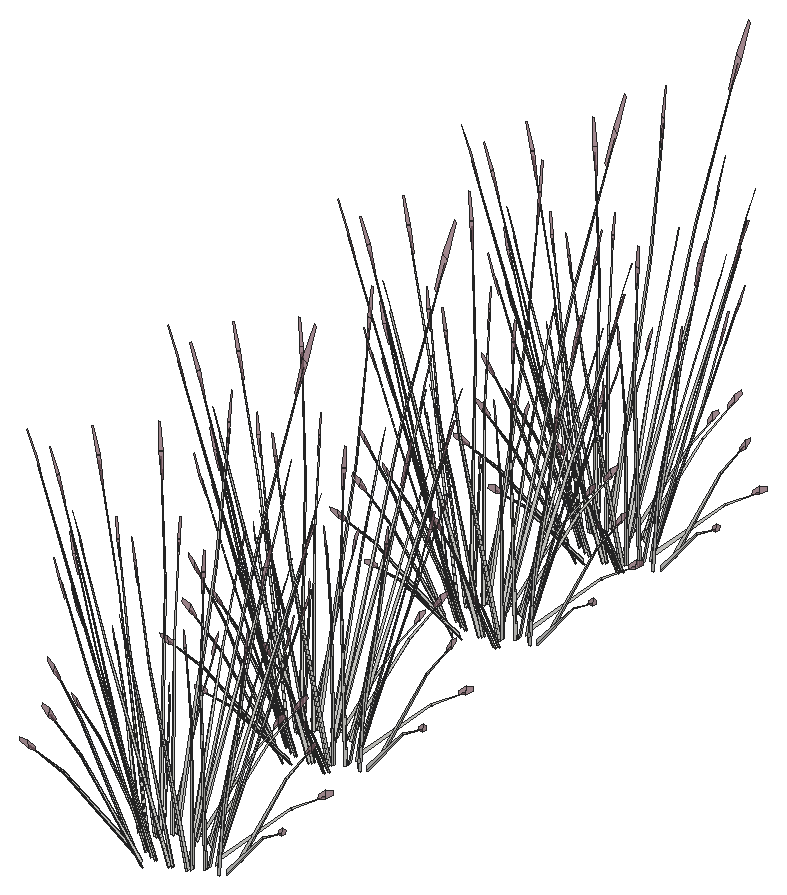
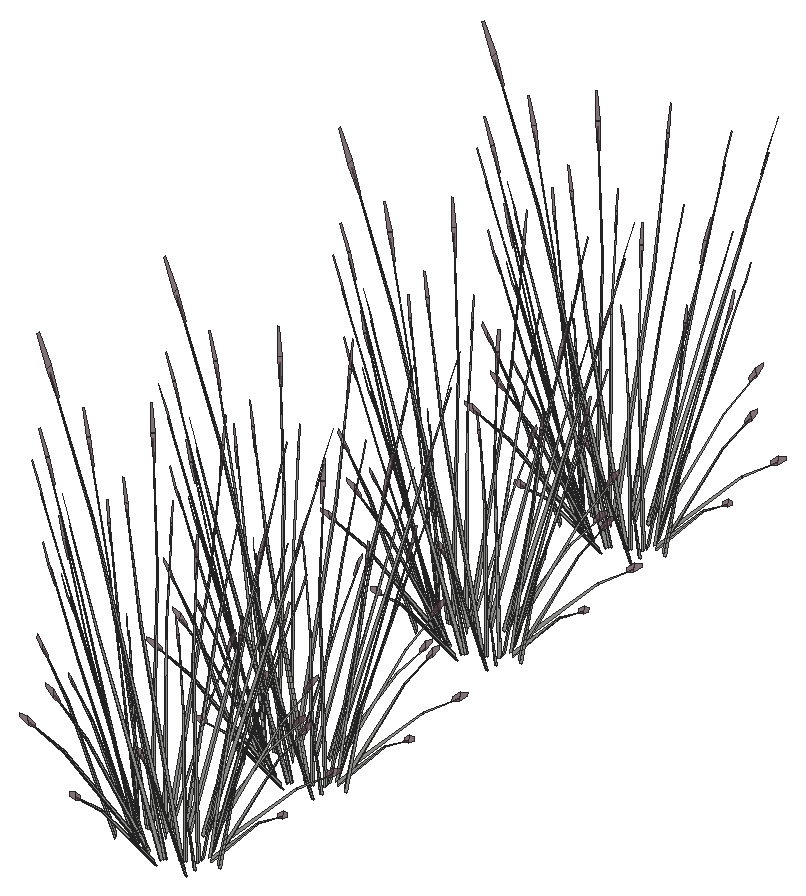
# SketchUp Ruby script. Lengths in inches.
U = 1.inch
M = Sketchup.active_model
def pt(a) = Geom::Point3d.new(a.map { |v| v * U })
def face(e, loops, mat)
  f = e.add_face(loops[0].map { |a| pt(a) })
  loops[1..].each { |l| e.add_face(l.map { |a| pt(a) }).erase! }
  f.material = f.back_material = mat if mat
  f
end
# faces: each face lists its corners as indices into pts; further lists are holes
def faces(e, pts, list, mat = nil) = list.each { |f| face(e, (f[0].is_a?(Array) ? f : [f]).map { |l| l.map { |i| pts[i] } }, mat) }
# xy, xz, yz: faces in a plane at the given z, y or x. An outline is a flat list of corners, or four numbers for a rectangle; further outlines are holes
def ring(l) = l.size == 4 ? [[l[0], l[1]], [l[2], l[1]], [l[2], l[3]], [l[0], l[3]]] : l.each_slice(2).to_a
def flat(e, list, mat, &to3) = list.each { |f| face(e, (f[0].is_a?(Array) ? f : [f]).map { |l| ring(l).map { |u, v| to3.(u, v) } }, mat) }
def xy(e, z, list, mat = nil) = flat(e, list, mat) { |x, y| [x, y, z] }
def xz(e, y, list, mat = nil) = flat(e, list, mat) { |x, z| [x, y, z] }
def yz(e, x, list, mat = nil) = flat(e, list, mat) { |y, z| [x, y, z] }
def lines(e, pts, list) = list.each { |a, b| e.add_line(pt(pts[a]), pt(pts[b])) }
# prism: a flat outline (further loops are holes) pulled along v
def prism(e, loops, v, mat = nil)
  f = face(e, loops, mat); d = Geom::Vector3d.new(v.map { |x| x * U })
  f.pushpull(f.normal.samedirection?(d) ? d.length : -d.length)
end
def box(e, o, s, mat = nil) = prism(e, [[o, [o[0] + s[0], o[1], o[2]], [o[0] + s[0], o[1] + s[1], o[2]], [o[0], o[1] + s[1], o[2]]]], [0, 0, s[2]], mat)
def at(x, y, z, deg = 0) = Geom::Transformation.translation(pt([x, y, z])) * Geom::Transformation.rotation(ORIGIN, Z_AXIS, deg.degrees)
def axes(o, x, y, z) = Geom::Transformation.new([*x, 0, *y, 0, *z, 0, *pt(o).to_a, 1])
def part(name) = M.definitions.add(name)
# library, detail: a bought-in or finely detailed component or shape, given as its bounding box
def library(name, o, s) = part(name).tap { |d| box(d.entities, o, s) }
def detail(e, o, s) = box(e.add_group.entities, o, s)
def put(e, d, t, mat = nil) = e.add_instance(d, t).tap { |i| i.material = mat if mat }
def group(e, t, mat = nil) = e.add_group.tap { |g| g.transformation = t; g.material = mat if mat }.entities
root = M.entities
M.materials.add("LightPink_Translucent").color = [144, 107, 117]
M.materials["LightPink_Translucent"].alpha = 0.75
c1 = part("blade")
p = [[2.15,0.21,22],[0,0.17,0],[0.09,0.45,0],[2.18,0.31,22],[2.29,0.31,22],[0.38,0.45,0],
  [2.48,0.24,33],[2.49,0.24,33],[2.48,0.22,33]]
faces(c1.entities,p,[[0,1,2,3],[4,5,2,3],[6,3,4,7],[8,0,3,6]])
c2 = part("seeds")
p = [[0.3,-0.1,1.38],[-0.01,-0.03,1.59],[-0.01,-0.03,0.03],[0.14,-0.07,-0.07],[0.29,-0.03,3],[0.15,0.01,3.11]]
faces(c2.entities,p,[[0,1,2,3],[1,0,4,5]],"LightPink_Translucent")
c3 = part("blade with seeds")
put(c3.entities,c1,at(0,0,0))
put(c3.entities,c2,axes([2.4,0.25,30.99],[1.5799,-0.05474,1.17369],[-0.12525,1.92788,0.29478],[-0.07173,-0.02425,1.56792]))
put(root,c3,axes([407.79,166.14,259.71],[-0.01417,0.07324,1.77383],[-0.6991,0.2658,-0.16761],[-0.20573,-0.13587,0.31391]))
put(root,c3,axes([409.76,167.74,260.03],[-0.74352,0.28449,-0.1216],[-0.36538,-0.50492,-0.67495],[-0.0981,-0.21277,1.02557]))
put(root,c3,axes([411.31,168.38,260.03],[-0.83505,-0.03027,-0.1216],[0.02282,-0.57322,-0.67495],[0.05801,-0.22077,1.02557]))
put(root,c3,axes([409.75,167.51,259.73],[0.55987,-0.20767,0.0643],[0.27403,0.37869,0.50621],[-0.05407,-0.16693,0.77189]))
put(root,c3,axes([407.83,167.57,259.73],[0.34533,-0.38816,0.0643],[0.49176,0.22599,0.50621],[-0.15898,-0.12445,0.77189]))
put(root,c3,axes([407.98,167.53,260.43],[-0.50709,0.58578,-0.13619],[-0.73436,-0.33748,-0.75594],[-0.25527,-0.1655,1.14864]))
put(root,c3,axes([411.45,168.18,259.73],[0.62439,0.02847,0.0643],[-0.01712,0.42991,0.50621],[0.06534,-0.16468,0.77189]))
put(root,c3,axes([406.04,167.36,259.72],[-0.16348,-0.00431,1.74944],[-0.52047,0.43131,-0.27667],[-0.2777,-0.08813,0.14031]))
put(root,c3,axes([412.22,169.51,260.03],[-0.70283,-0.33692,-0.1216],[0.40491,-0.48793,-0.67495],[0.19857,-0.16961,1.02557]))
put(root,c3,axes([413.95,169.36,259.71],[-0.09924,-0.00464,1.77383],[-0.4121,-0.49725,-0.16761],[0.1655,-0.1635,0.31391]))
put(root,c3,axes([406.21,168.33,259.73],[0.03826,-0.46465,0.0643],[0.57772,0.01274,0.50621],[-0.2213,-0.04862,0.77189]))
put(root,c3,axes([412.47,169.38,259.73],[0.52161,0.25698,0.0643],[-0.30368,0.36595,0.50621],[0.16723,-0.11831,0.77189]))
put(root,c3,axes([414.32,169.96,259.72],[0.10543,-0.09307,1.74944],[-0.13495,-0.57092,-0.27667],[0.26455,-0.10825,0.14031]))
put(root,c3,axes([405.41,167.73,259.71],[0.05633,0.06098,1.77383],[-0.27155,0.54815,-0.16761],[-0.27501,0.00397,0.31391]))
put(root,c3,axes([406.48,168.4375,260.03],[-0.04068,0.62141,-0.1216],[-0.77029,-0.01698,-0.67495],[-0.29667,-0.04317,1.02557]))
put(root,c3,axes([412.24,170.82,260.03],[-0.38229,-0.5533,-0.1216],[0.6785,-0.2719,-0.67495],[0.28593,-0.073,1.02557]))
put(root,c3,axes([405.31,169.6,259.73],[-0.27906,-0.41663,0.0643],[0.50888,-0.20393,0.50621],[-0.22432,0.04024,0.77189]))
put(root,c3,axes([412.55,170.8125,259.73],[0.27906,0.41663,0.0643],[-0.50888,0.20393,0.50621],[0.22432,-0.04024,0.77189]))
put(root,c3,axes([413.76,172.47,259.71],[-0.0687,-0.05349,1.77383],[0.15029,-0.57341,-0.16761],[0.27062,-0.03664,0.31391]))
put(root,c3,axes([404.82,170.14,259.72],[-0.12407,0.07933,1.74944],[0.01055,0.57963,-0.27667],[-0.2844,0.07538,0.14031]))
put(root,c3,axes([405.62,169.59,260.03],[0.38229,0.5533,-0.1216],[-0.6785,0.2719,-0.67495],[-0.28593,0.073,1.02557]))
put(root,c3,axes([411.39,171.97,260.03],[0.04068,-0.62141,-0.1216],[0.77029,0.01698,-0.67495],[0.29667,0.04317,1.02557]))
put(root,c3,axes([412.06,171.6,259.72],[0.16299,-0.01033,1.74944],[0.44707,-0.47471,-0.27667],[0.28992,0.06266,0.14031]))
put(root,c3,axes([405.39,171.03,259.73],[-0.52161,-0.25698,0.0643],[0.30368,-0.36595,0.50621],[-0.16723,0.11831,0.77189]))
put(root,c3,axes([403.44,170.73,259.71],[0.09697,0.01639,1.77383],[0.29997,0.53988,-0.16761],[-0.1985,0.1417,0.31391]))
put(root,c3,axes([411.66,172.08,259.73],[-0.03826,0.46465,0.0643],[-0.57772,-0.01274,0.50621],[0.2213,0.04862,0.77189]))
put(root,c3,axes([410.38,169.5625,259.47],[-0.65655,-0.31748,1.38283],[0.69326,-0.49431,0.59665],[0.21183,0.29789,1.33663]))
put(root,c3,axes([405.65,170.9,260.03],[0.70283,0.33692,-0.1216],[-0.40491,0.48793,-0.67495],[-0.19857,0.16961,1.02557]))
put(root,c3,axes([409.87,172.65,260.03],[0.45276,-0.52302,-0.1216],[0.65568,0.30132,-0.67495],[0.22792,0.14777,1.02557]))
put(root,c3,axes([409.28,173.08,259.71],[0.00225,-0.07398,1.77383],[0.65113,-0.32638,-0.16761],[0.22617,0.1165,0.31391]))
put(root,c3,axes([406.42,172.23,259.73],[-0.62439,-0.02847,0.0643],[0.01712,-0.42991,0.50621],[-0.06534,0.16468,0.77189]))
put(root,c3,axes([410.04,172.84,259.73],[-0.34533,0.38816,0.0643],[-0.49176,-0.22599,0.50621],[0.15898,0.12445,0.77189]))
put(root,c3,axes([408.12,172.9,259.73],[-0.55987,0.20767,0.0643],[-0.27403,-0.37869,0.50621],[0.05407,0.16693,0.77189]))
put(root,c3,axes([404.84,172.3,259.72],[-0.01889,0.12092,1.74944],[0.53598,0.42065,-0.27667],[-0.14032,0.19892,0.14031]))
put(root,c3,axes([406.56,172.03,260.4],[0.83505,0.03027,-0.13498],[-0.02282,0.57322,-0.74919],[-0.05801,0.22077,1.13838]))
put(root,c3,axes([408.1,172.67,260.03],[0.74352,-0.28449,-0.1216],[0.36538,0.50492,-0.67495],[0.0981,0.21277,1.02557]))
put(root,c3,axes([404.78,173.54,259.71],[0.0862,-0.03689,1.77383],[0.71245,0.24539,-0.16761],[-0.01674,0.20431,0.31391]))
put(root,c3,axes([407.93,173.8,259.72],[0.09631,0.0984,1.74944],[0.77725,0.03866,-0.27667],[0.07816,0.217,0.14031]))
put(root,c3,axes([406.5625,188.55,259.72],[-0.11621,-0.08567,1.74944],[-0.77555,0.05431,-0.27667],[-0.12378,-0.20491,0.14031]))
put(root,c3,axes([410.05,189.6,259.72],[-0.00733,-0.12161,1.74944],[-0.61946,-0.35147,-0.27667],[0.09577,-0.21306,0.14031]))
put(root,c3,axes([409.88,189.16,259.71],[-0.07716,0.04667,1.77383],[-0.75601,-0.15746,-0.16761],[-0.02737,-0.20368,0.31391]))
put(root,c3,axes([405.77,188.27,259.71],[-0.01417,0.07324,1.77383],[-0.6991,0.2658,-0.16761],[-0.20573,-0.13587,0.31391]))
put(root,c3,axes([407.74,189.87,260.03],[-0.74352,0.28449,-0.1216],[-0.36538,-0.50492,-0.67495],[-0.0981,-0.21277,1.02557]))
put(root,c3,axes([409.29,190.51,260.03],[-0.83505,-0.03027,-0.1216],[0.02282,-0.57322,-0.67495],[0.05801,-0.22077,1.02557]))
put(root,c3,axes([407.73,189.64,259.73],[0.55987,-0.20767,0.0643],[0.27403,0.37869,0.50621],[-0.05407,-0.16693,0.77189]))
put(root,c3,axes([405.81,189.7,259.73],[0.34533,-0.38816,0.0643],[0.49176,0.22599,0.50621],[-0.15898,-0.12445,0.77189]))
put(root,c3,axes([405.96,189.66,260.43],[-0.50709,0.58578,-0.13619],[-0.73436,-0.33748,-0.75594],[-0.25527,-0.1655,1.14864]))
put(root,c3,axes([409.43,190.31,259.73],[0.62439,0.02847,0.0643],[-0.01712,0.42991,0.50621],[0.06534,-0.16468,0.77189]))
put(root,c3,axes([404.02,189.49,259.72],[-0.16348,-0.00431,1.74944],[-0.52047,0.43131,-0.27667],[-0.2777,-0.08813,0.14031]))
put(root,c3,axes([410.2,191.64,260.03],[-0.70283,-0.33692,-0.1216],[0.40491,-0.48793,-0.67495],[0.19857,-0.16961,1.02557]))
put(root,c3,axes([411.93,191.49,259.71],[-0.09924,-0.00464,1.77383],[-0.4121,-0.49725,-0.16761],[0.1655,-0.1635,0.31391]))
put(root,c3,axes([404.1875,190.47,259.73],[0.03826,-0.46465,0.0643],[0.57772,0.01274,0.50621],[-0.2213,-0.04862,0.77189]))
put(root,c3,axes([410.45,191.51,259.73],[0.52161,0.25698,0.0643],[-0.30368,0.36595,0.50621],[0.16723,-0.11831,0.77189]))
put(root,c3,axes([412.3,192.09,259.72],[0.10543,-0.09307,1.74944],[-0.13495,-0.57092,-0.27667],[0.26455,-0.10825,0.14031]))
put(root,c3,axes([403.39,189.86,259.71],[0.05633,0.06098,1.77383],[-0.27155,0.54815,-0.16761],[-0.27501,0.00397,0.31391]))
put(root,c3,axes([404.46,190.57,260.03],[-0.04068,0.62141,-0.1216],[-0.77029,-0.01698,-0.67495],[-0.29667,-0.04317,1.02557]))
put(root,c3,axes([410.23,192.95,260.03],[-0.38229,-0.5533,-0.1216],[0.6785,-0.2719,-0.67495],[0.28593,-0.073,1.02557]))
put(root,c3,axes([403.3,191.73,259.73],[-0.27906,-0.41663,0.0643],[0.50888,-0.20393,0.50621],[-0.22432,0.04024,0.77189]))
put(root,c3,axes([410.53,192.94,259.73],[0.27906,0.41663,0.0643],[-0.50888,0.20393,0.50621],[0.22432,-0.04024,0.77189]))
put(root,c3,axes([411.75,194.6,259.71],[-0.0687,-0.05349,1.77383],[0.15029,-0.57341,-0.16761],[0.27062,-0.03664,0.31391]))
put(root,c3,axes([402.8,192.27,259.72],[-0.12407,0.07933,1.74944],[0.01055,0.57963,-0.27667],[-0.2844,0.07538,0.14031]))
put(root,c3,axes([403.6,191.72,260.03],[0.38229,0.5533,-0.1216],[-0.6785,0.2719,-0.67495],[-0.28593,0.073,1.02557]))
put(root,c3,axes([409.37,194.1,260.03],[0.04068,-0.62141,-0.1216],[0.77029,0.01698,-0.67495],[0.29667,0.04317,1.02557]))
put(root,c3,axes([410.04,193.73,259.72],[0.16299,-0.01033,1.74944],[0.44707,-0.47471,-0.27667],[0.28992,0.06266,0.14031]))
put(root,c3,axes([403.375,193.16,259.73],[-0.52161,-0.25698,0.0643],[0.30368,-0.36595,0.50621],[-0.16723,0.11831,0.77189]))
put(root,c3,axes([401.43,192.86,259.71],[0.09697,0.01639,1.77383],[0.29997,0.53988,-0.16761],[-0.1985,0.1417,0.31391]))
put(root,c3,axes([409.64,194.21,259.73],[-0.03826,0.46465,0.0643],[-0.57772,-0.01274,0.50621],[0.2213,0.04862,0.77189]))
put(root,c3,axes([408.36,191.69,259.47],[-0.65655,-0.31748,1.38283],[0.69326,-0.49431,0.59665],[0.21183,0.29789,1.33663]))
put(root,c3,axes([403.63,193.03,260.03],[0.70283,0.33692,-0.1216],[-0.40491,0.48793,-0.67495],[-0.19857,0.16961,1.02557]))
put(root,c3,axes([407.85,194.78,260.03],[0.45276,-0.52302,-0.1216],[0.65568,0.30132,-0.67495],[0.22792,0.14777,1.02557]))
put(root,c3,axes([407.26,195.21,259.71],[0.00225,-0.07398,1.77383],[0.65113,-0.32638,-0.16761],[0.22617,0.1165,0.31391]))
put(root,c3,axes([404.4,194.37,259.73],[-0.62439,-0.02847,0.0643],[0.01712,-0.42991,0.50621],[-0.06534,0.16468,0.77189]))
put(root,c3,axes([408.02,194.97,259.73],[-0.34533,0.38816,0.0643],[-0.49176,-0.22599,0.50621],[0.15898,0.12445,0.77189]))
put(root,c3,axes([406.1,195.03,259.73],[-0.55987,0.20767,0.0643],[-0.27403,-0.37869,0.50621],[0.05407,0.16693,0.77189]))
put(root,c3,axes([402.82,194.43,259.72],[-0.01889,0.12092,1.74944],[0.53598,0.42065,-0.27667],[-0.14032,0.19892,0.14031]))
put(root,c3,axes([404.54,194.16,260.4],[0.83505,0.03027,-0.13498],[-0.02282,0.57322,-0.74919],[-0.05801,0.22077,1.13838]))
put(root,c3,axes([406.08,194.8,260.03],[0.74352,-0.28449,-0.1216],[0.36538,0.50492,-0.67495],[0.0981,0.21277,1.02557]))
put(root,c3,axes([402.76,195.67,259.71],[0.0862,-0.03689,1.77383],[0.71245,0.24539,-0.16761],[-0.01674,0.20431,0.31391]))
put(root,c3,axes([405.91,195.93,259.72],[0.09631,0.0984,1.74944],[0.77725,0.03866,-0.27667],[0.07816,0.217,0.14031]))
put(root,c3,axes([404.16,215.3,259.72],[-0.11621,-0.08567,1.74944],[-0.77555,0.05431,-0.27667],[-0.12378,-0.20491,0.14031]))
put(root,c3,axes([407.64,216.35,259.72],[-0.00733,-0.12161,1.74944],[-0.61946,-0.35147,-0.27667],[0.09577,-0.21306,0.14031]))
put(root,c3,axes([407.48,215.92,259.71],[-0.07716,0.04667,1.77383],[-0.75601,-0.15746,-0.16761],[-0.02737,-0.20368,0.31391]))
put(root,c3,axes([403.37,215.02,259.71],[-0.01417,0.07324,1.77383],[-0.6991,0.2658,-0.16761],[-0.20573,-0.13587,0.31391]))
put(root,c3,axes([405.34,216.625,260.03],[-0.74352,0.28449,-0.1216],[-0.36538,-0.50492,-0.67495],[-0.0981,-0.21277,1.02557]))
put(root,c3,axes([406.89,217.26,260.03],[-0.83505,-0.03027,-0.1216],[0.02282,-0.57322,-0.67495],[0.05801,-0.22077,1.02557]))
put(root,c3,axes([405.32,216.4,259.73],[0.55987,-0.20767,0.0643],[0.27403,0.37869,0.50621],[-0.05407,-0.16693,0.77189]))
put(root,c3,axes([403.41,216.46,259.73],[0.34533,-0.38816,0.0643],[0.49176,0.22599,0.50621],[-0.15898,-0.12445,0.77189]))
put(root,c3,axes([403.5625,216.42,260.43],[-0.50709,0.58578,-0.13619],[-0.73436,-0.33748,-0.75594],[-0.25527,-0.1655,1.14864]))
put(root,c3,axes([407.02,217.0625,259.73],[0.62439,0.02847,0.0643],[-0.01712,0.42991,0.50621],[0.06534,-0.16468,0.77189]))
put(root,c3,axes([401.62,216.25,259.72],[-0.16348,-0.00431,1.74944],[-0.52047,0.43131,-0.27667],[-0.2777,-0.08813,0.14031]))
put(root,c3,axes([407.79,218.39,260.03],[-0.70283,-0.33692,-0.1216],[0.40491,-0.48793,-0.67495],[0.19857,-0.16961,1.02557]))
put(root,c3,axes([409.52,218.25,259.71],[-0.09924,-0.00464,1.77383],[-0.4121,-0.49725,-0.16761],[0.1655,-0.1635,0.31391]))
put(root,c3,axes([401.78,217.22,259.73],[0.03826,-0.46465,0.0643],[0.57772,0.01274,0.50621],[-0.2213,-0.04862,0.77189]))
put(root,c3,axes([408.05,218.27,259.73],[0.52161,0.25698,0.0643],[-0.30368,0.36595,0.50621],[0.16723,-0.11831,0.77189]))
put(root,c3,axes([409.9,218.84,259.72],[0.10543,-0.09307,1.74944],[-0.13495,-0.57092,-0.27667],[0.26455,-0.10825,0.14031]))
put(root,c3,axes([400.99,216.61,259.71],[0.05633,0.06098,1.77383],[-0.27155,0.54815,-0.16761],[-0.27501,0.00397,0.31391]))
put(root,c3,axes([402.06,217.32,260.03],[-0.04068,0.62141,-0.1216],[-0.77029,-0.01698,-0.67495],[-0.29667,-0.04317,1.02557]))
put(root,c3,axes([407.82,219.71,260.03],[-0.38229,-0.5533,-0.1216],[0.6785,-0.2719,-0.67495],[0.28593,-0.073,1.02557]))
put(root,c3,axes([400.89,218.48,259.73],[-0.27906,-0.41663,0.0643],[0.50888,-0.20393,0.50621],[-0.22432,0.04024,0.77189]))
put(root,c3,axes([408.13,219.7,259.73],[0.27906,0.41663,0.0643],[-0.50888,0.20393,0.50621],[0.22432,-0.04024,0.77189]))
put(root,c3,axes([409.34,221.35,259.71],[-0.0687,-0.05349,1.77383],[0.15029,-0.57341,-0.16761],[0.27062,-0.03664,0.31391]))
put(root,c3,axes([400.4,219.03,259.72],[-0.12407,0.07933,1.74944],[0.01055,0.57963,-0.27667],[-0.2844,0.07538,0.14031]))
put(root,c3,axes([401.2,218.47,260.03],[0.38229,0.5533,-0.1216],[-0.6785,0.2719,-0.67495],[-0.28593,0.073,1.02557]))
put(root,c3,axes([406.96,220.86,260.03],[0.04068,-0.62141,-0.1216],[0.77029,0.01698,-0.67495],[0.29667,0.04317,1.02557]))
put(root,c3,axes([407.63,220.48,259.72],[0.16299,-0.01033,1.74944],[0.44707,-0.47471,-0.27667],[0.28992,0.06266,0.14031]))
put(root,c3,axes([400.97,219.91,259.73],[-0.52161,-0.25698,0.0643],[0.30368,-0.36595,0.50621],[-0.16723,0.11831,0.77189]))
put(root,c3,axes([399.02,219.61,259.71],[0.09697,0.01639,1.77383],[0.29997,0.53988,-0.16761],[-0.1985,0.1417,0.31391]))
put(root,c3,axes([407.24,220.96,259.73],[-0.03826,0.46465,0.0643],[-0.57772,-0.01274,0.50621],[0.2213,0.04862,0.77189]))
put(root,c3,axes([405.96,218.45,259.47],[-0.65655,-0.31748,1.38283],[0.69326,-0.49431,0.59665],[0.21183,0.29789,1.33663]))
put(root,c3,axes([401.23,219.79,260.03],[0.70283,0.33692,-0.1216],[-0.40491,0.48793,-0.67495],[-0.19857,0.16961,1.02557]))
put(root,c3,axes([405.45,221.53,260.03],[0.45276,-0.52302,-0.1216],[0.65568,0.30132,-0.67495],[0.22792,0.14777,1.02557]))
put(root,c3,axes([404.85,221.97,259.71],[0.00225,-0.07398,1.77383],[0.65113,-0.32638,-0.16761],[0.22617,0.1165,0.31391]))
put(root,c3,axes([402,221.12,259.73],[-0.62439,-0.02847,0.0643],[0.01712,-0.42991,0.50621],[-0.06534,0.16468,0.77189]))
put(root,c3,axes([405.62,221.72,259.73],[-0.34533,0.38816,0.0643],[-0.49176,-0.22599,0.50621],[0.15898,0.12445,0.77189]))
put(root,c3,axes([403.7,221.78,259.73],[-0.55987,0.20767,0.0643],[-0.27403,-0.37869,0.50621],[0.05407,0.16693,0.77189]))
put(root,c3,axes([400.42,221.1875,259.72],[-0.01889,0.12092,1.74944],[0.53598,0.42065,-0.27667],[-0.14032,0.19892,0.14031]))
put(root,c3,axes([402.14,220.92,260.4],[0.83505,0.03027,-0.13498],[-0.02282,0.57322,-0.74919],[-0.05801,0.22077,1.13838]))
put(root,c3,axes([403.68,221.55,260.03],[0.74352,-0.28449,-0.1216],[0.36538,0.50492,-0.67495],[0.0981,0.21277,1.02557]))
put(root,c3,axes([400.36,222.43,259.71],[0.0862,-0.03689,1.77383],[0.71245,0.24539,-0.16761],[-0.01674,0.20431,0.31391]))
put(root,c3,axes([403.51,222.68,259.72],[0.09631,0.0984,1.74944],[0.77725,0.03866,-0.27667],[0.07816,0.217,0.14031]))
put(root,c3,axes([404.32,232.375,259.72],[-0.11621,-0.08567,1.74944],[-0.77555,0.05431,-0.27667],[-0.12378,-0.20491,0.14031]))
put(root,c3,axes([407.8,233.42,259.72],[-0.00733,-0.12161,1.74944],[-0.61946,-0.35147,-0.27667],[0.09577,-0.21306,0.14031]))
put(root,c3,axes([407.64,232.99,259.71],[-0.07716,0.04667,1.77383],[-0.75601,-0.15746,-0.16761],[-0.02737,-0.20368,0.31391]))
put(root,c3,axes([403.52,232.09,259.71],[-0.01417,0.07324,1.77383],[-0.6991,0.2658,-0.16761],[-0.20573,-0.13587,0.31391]))
put(root,c3,axes([405.5,233.7,260.03],[-0.74352,0.28449,-0.1216],[-0.36538,-0.50492,-0.67495],[-0.0981,-0.21277,1.02557]))
put(root,c3,axes([407.04,234.34,260.03],[-0.83505,-0.03027,-0.1216],[0.02282,-0.57322,-0.67495],[0.05801,-0.22077,1.02557]))
put(root,c3,axes([405.48,233.47,259.73],[0.55987,-0.20767,0.0643],[0.27403,0.37869,0.50621],[-0.05407,-0.16693,0.77189]))
put(root,c3,axes([403.56,233.53,259.73],[0.34533,-0.38816,0.0643],[0.49176,0.22599,0.50621],[-0.15898,-0.12445,0.77189]))
put(root,c3,axes([403.72,233.49,260.43],[-0.50709,0.58578,-0.13619],[-0.73436,-0.33748,-0.75594],[-0.25527,-0.1655,1.14864]))
put(root,c3,axes([407.18,234.13,259.73],[0.62439,0.02847,0.0643],[-0.01712,0.42991,0.50621],[0.06534,-0.16468,0.77189]))
put(root,c3,axes([401.78,233.32,259.72],[-0.16348,-0.00431,1.74944],[-0.52047,0.43131,-0.27667],[-0.2777,-0.08813,0.14031]))
put(root,c3,axes([407.95,235.46,260.03],[-0.70283,-0.33692,-0.1216],[0.40491,-0.48793,-0.67495],[0.19857,-0.16961,1.02557]))
put(root,c3,axes([409.68,235.32,259.71],[-0.09924,-0.00464,1.77383],[-0.4121,-0.49725,-0.16761],[0.1655,-0.1635,0.31391]))
put(root,c3,axes([401.94,234.29,259.73],[0.03826,-0.46465,0.0643],[0.57772,0.01274,0.50621],[-0.2213,-0.04862,0.77189]))
put(root,c3,axes([408.21,235.34,259.73],[0.52161,0.25698,0.0643],[-0.30368,0.36595,0.50621],[0.16723,-0.11831,0.77189]))
put(root,c3,axes([410.06,235.91,259.72],[0.10543,-0.09307,1.74944],[-0.13495,-0.57092,-0.27667],[0.26455,-0.10825,0.14031]))
put(root,c3,axes([401.15,233.68,259.71],[0.05633,0.06098,1.77383],[-0.27155,0.54815,-0.16761],[-0.27501,0.00397,0.31391]))
put(root,c3,axes([402.22,234.39,260.03],[-0.04068,0.62141,-0.1216],[-0.77029,-0.01698,-0.67495],[-0.29667,-0.04317,1.02557]))
put(root,c3,axes([407.98,236.78,260.03],[-0.38229,-0.5533,-0.1216],[0.6785,-0.2719,-0.67495],[0.28593,-0.073,1.02557]))
put(root,c3,axes([401.05,235.56,259.73],[-0.27906,-0.41663,0.0643],[0.50888,-0.20393,0.50621],[-0.22432,0.04024,0.77189]))
put(root,c3,axes([408.29,236.77,259.73],[0.27906,0.41663,0.0643],[-0.50888,0.20393,0.50621],[0.22432,-0.04024,0.77189]))
put(root,c3,axes([409.5,238.42,259.71],[-0.0687,-0.05349,1.77383],[0.15029,-0.57341,-0.16761],[0.27062,-0.03664,0.31391]))
put(root,c3,axes([400.56,236.1,259.72],[-0.12407,0.07933,1.74944],[0.01055,0.57963,-0.27667],[-0.2844,0.07538,0.14031]))
put(root,c3,axes([401.36,235.54,260.03],[0.38229,0.5533,-0.1216],[-0.6785,0.2719,-0.67495],[-0.28593,0.073,1.02557]))
put(root,c3,axes([407.12,237.93,260.03],[0.04068,-0.62141,-0.1216],[0.77029,0.01698,-0.67495],[0.29667,0.04317,1.02557]))
put(root,c3,axes([407.79,237.56,259.72],[0.16299,-0.01033,1.74944],[0.44707,-0.47471,-0.27667],[0.28992,0.06266,0.14031]))
put(root,c3,axes([401.13,236.98,259.73],[-0.52161,-0.25698,0.0643],[0.30368,-0.36595,0.50621],[-0.16723,0.11831,0.77189]))
put(root,c3,axes([399.18,236.68,259.71],[0.09697,0.01639,1.77383],[0.29997,0.53988,-0.16761],[-0.1985,0.1417,0.31391]))
put(root,c3,axes([407.4,238.03,259.73],[-0.03826,0.46465,0.0643],[-0.57772,-0.01274,0.50621],[0.2213,0.04862,0.77189]))
put(root,c3,axes([406.12,235.52,259.47],[-0.65655,-0.31748,1.38283],[0.69326,-0.49431,0.59665],[0.21183,0.29789,1.33663]))
put(root,c3,axes([401.39,236.86,260.03],[0.70283,0.33692,-0.1216],[-0.40491,0.48793,-0.67495],[-0.19857,0.16961,1.02557]))
put(root,c3,axes([405.61,238.6,260.03],[0.45276,-0.52302,-0.1216],[0.65568,0.30132,-0.67495],[0.22792,0.14777,1.02557]))
put(root,c3,axes([405.01,239.04,259.71],[0.00225,-0.07398,1.77383],[0.65113,-0.32638,-0.16761],[0.22617,0.1165,0.31391]))
put(root,c3,axes([402.16,238.19,259.73],[-0.62439,-0.02847,0.0643],[0.01712,-0.42991,0.50621],[-0.06534,0.16468,0.77189]))
put(root,c3,axes([405.77,238.8,259.73],[-0.34533,0.38816,0.0643],[-0.49176,-0.22599,0.50621],[0.15898,0.12445,0.77189]))
put(root,c3,axes([403.86,238.85,259.73],[-0.55987,0.20767,0.0643],[-0.27403,-0.37869,0.50621],[0.05407,0.16693,0.77189]))
put(root,c3,axes([400.58,238.26,259.72],[-0.01889,0.12092,1.74944],[0.53598,0.42065,-0.27667],[-0.14032,0.19892,0.14031]))
put(root,c3,axes([402.29,237.99,260.4],[0.83505,0.03027,-0.13498],[-0.02282,0.57322,-0.74919],[-0.05801,0.22077,1.13838]))
put(root,c3,axes([403.84,238.625,260.03],[0.74352,-0.28449,-0.1216],[0.36538,0.50492,-0.67495],[0.0981,0.21277,1.02557]))
put(root,c3,axes([400.52,239.5,259.71],[0.0862,-0.03689,1.77383],[0.71245,0.24539,-0.16761],[-0.01674,0.20431,0.31391]))
put(root,c3,axes([403.66,239.76,259.72],[0.09631,0.0984,1.74944],[0.77725,0.03866,-0.27667],[0.07816,0.217,0.14031]))
